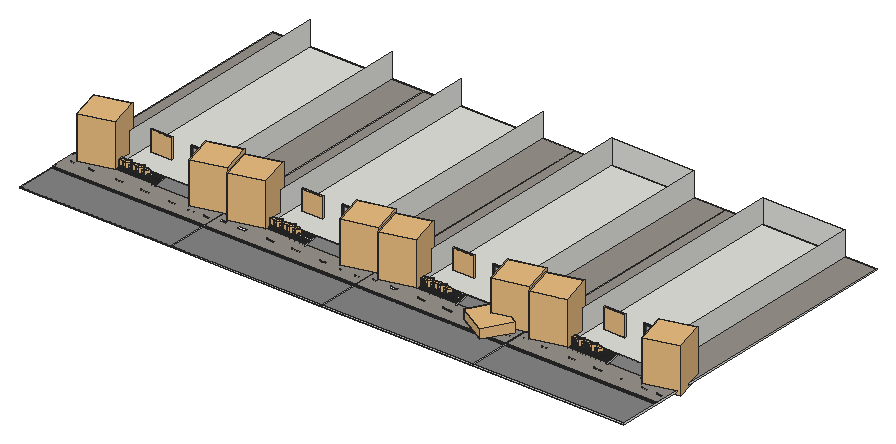
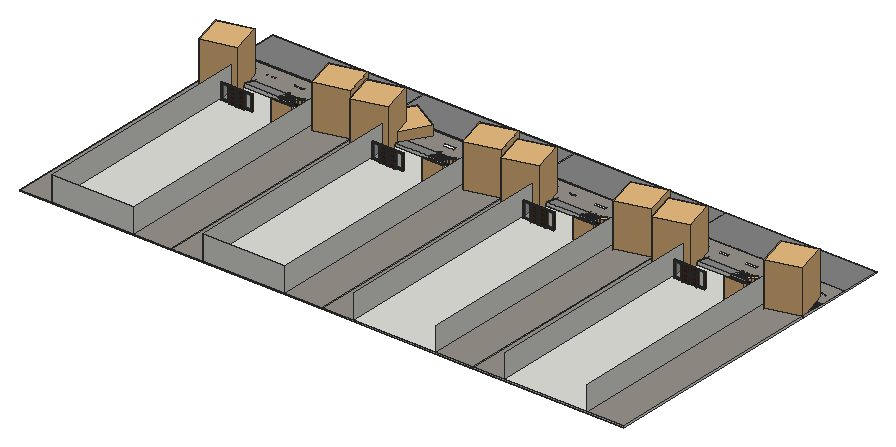
# SketchUp Ruby script. Lengths in inches.
U = 1.inch
M = Sketchup.active_model
def pt(a) = Geom::Point3d.new(a.map { |v| v * U })
def face(e, loops, mat)
  f = e.add_face(loops[0].map { |a| pt(a) })
  loops[1..].each { |l| e.add_face(l.map { |a| pt(a) }).erase! }
  f.material = f.back_material = mat if mat
  f
end
# faces: each face lists its corners as indices into pts; further lists are holes
def faces(e, pts, list, mat = nil) = list.each { |f| face(e, (f[0].is_a?(Array) ? f : [f]).map { |l| l.map { |i| pts[i] } }, mat) }
# xy, xz, yz: faces in a plane at the given z, y or x. An outline is a flat list of corners, or four numbers for a rectangle; further outlines are holes
def ring(l) = l.size == 4 ? [[l[0], l[1]], [l[2], l[1]], [l[2], l[3]], [l[0], l[3]]] : l.each_slice(2).to_a
def flat(e, list, mat, &to3) = list.each { |f| face(e, (f[0].is_a?(Array) ? f : [f]).map { |l| ring(l).map { |u, v| to3.(u, v) } }, mat) }
def xy(e, z, list, mat = nil) = flat(e, list, mat) { |x, y| [x, y, z] }
def xz(e, y, list, mat = nil) = flat(e, list, mat) { |x, z| [x, y, z] }
def yz(e, x, list, mat = nil) = flat(e, list, mat) { |y, z| [x, y, z] }
def lines(e, pts, list) = list.each { |a, b| e.add_line(pt(pts[a]), pt(pts[b])) }
# prism: a flat outline (further loops are holes) pulled along v
def prism(e, loops, v, mat = nil)
  f = face(e, loops, mat); d = Geom::Vector3d.new(v.map { |x| x * U })
  f.pushpull(f.normal.samedirection?(d) ? d.length : -d.length)
end
def box(e, o, s, mat = nil) = prism(e, [[o, [o[0] + s[0], o[1], o[2]], [o[0] + s[0], o[1] + s[1], o[2]], [o[0], o[1] + s[1], o[2]]]], [0, 0, s[2]], mat)
def at(x, y, z, deg = 0) = Geom::Transformation.translation(pt([x, y, z])) * Geom::Transformation.rotation(ORIGIN, Z_AXIS, deg.degrees)
def axes(o, x, y, z) = Geom::Transformation.new([*x, 0, *y, 0, *z, 0, *pt(o).to_a, 1])
def part(name) = M.definitions.add(name)
# library, detail: a bought-in or finely detailed component or shape, given as its bounding box
def library(name, o, s) = part(name).tap { |d| box(d.entities, o, s) }
def detail(e, o, s) = box(e.add_group.entities, o, s)
def put(e, d, t, mat = nil) = e.add_instance(d, t).tap { |i| i.material = mat if mat }
def group(e, t, mat = nil) = e.add_group.tap { |g| g.transformation = t; g.material = mat if mat }.entities
root = M.entities
M.materials.add("Color_000").color = [255, 255, 255]
M.materials.add("MADEIRAS PORTAS MOD 4").color = [48, 37, 30]
M.materials.add("Material__1").color = [95, 70, 46]
M.materials.add("[Aluminum]").color = [179, 179, 179]
M.materials.add("[Color M07]").color = [58, 58, 58]
M.materials.add("[Color M08]").color = [30, 30, 30]
M.materials.add("[Granite Dark Gray]").color = [38, 37, 37]
M.materials.add("[Granite Tile]").color = [153, 146, 141]
M.materials.add("[Tile Grey]").color = [132, 132, 132]
M.materials.add("[Tile Grey]1").color = [133, 133, 133]
M.materials.add("[Translucent Glass Gray]").color = [128, 128, 128]
M.materials["[Translucent Glass Gray]"].alpha = 0.5
M.materials.add("[Wood Veneer 01]").color = [66, 38, 20]
c1 = library("002+Bmw+M4+++mat3.4+2017",[-252.8,19.48,9.01],[196.94,171.32,55.15])
c2 = part("Untitled (5)")
xy(c2.entities,0,[[[158.81,26.5625,306.06,993.3125],[226.57,518.17,239.57,583.92],[225.28,357.51,237.28,411.51],[222.61,182.28,236.36,226.53],[239.71,931.55,251.46,972.3],[233.64,703.93,242.14,755.18],[240.05,835.03,248.8,880.53],[222.04,66.5,231.29,100.5]]])
xy(c2.entities,0,[[222.04,66.5,231.29,100.5],[222.61,182.28,236.36,226.53],[225.28,357.51,237.28,411.51],[226.57,518.17,239.57,583.92],[233.64,703.93,242.14,755.18],
  [240.05,835.03,248.8,880.53],[239.71,931.55,251.46,972.3]],"Color_000")
c3 = library("Areca palm plant",[0,0,0],[49.1,36.6,54.46])
c4 = library("Group\#74",[-84.69,-90.07,-0.36],[176.51,175.13,171.4])
c5 = library("Group38\#2",[14.01,28.44,-23.43],[18.58,18.32,38.89])
c6 = library("Group\#130",[-7.34,-1.2,0],[38.67,35.81,49.04])
c7 = library("Group20\#1",[-20.81,-17.08,3.79],[39.86,39.43,37.51])
c8 = part("Group\#3")
xy(c8.entities,0,[[0,0,6,234.8],[30,0,36,234.8]])
xy(c8.entities,3,[[6,0,30,234.8]])
xy(c8.entities,7,[[6,5,30,229.8]],"Material__1")
xy(c8.entities,15,[[[0,0,36,234.8],[6,5,30,229.8]]])
xz(c8.entities,0,[[0,0,6,0,6,3,30,3,30,0,36,0,36,15,0,15]])
xz(c8.entities,5,[[6,7,30,15]])
xz(c8.entities,229.8,[[6,7,30,15]])
xz(c8.entities,234.8,[[0,0,0,15,36,15,36,0,30,0,30,3,6,3,6,0]])
yz(c8.entities,0,[[0,0,234.8,15]])
yz(c8.entities,6,[[0,0,234.8,3],[5,7,229.8,15]])
yz(c8.entities,30,[[0,0,234.8,3],[5,7,229.8,15]])
yz(c8.entities,36,[[0,0,234.8,15]])
c9 = part("Planted trough")
put(c9.entities,c3,axes([-6.2,158.41,6.08],[0.45017,-0.56191,0],[0.66137,0.52986,0],[0,0,0.72]))
put(c9.entities,c3,axes([-6.2,56.6,6.08],[0.45017,-0.56191,0],[0.66137,0.52986,0],[0,0,0.72]))
put(c9.entities,c4,axes([17.19,15.79,6.07],[-0.08133,-0.14087,0],[0.14087,-0.08133,0],[0,0,0.1725]))
put(c9.entities,c4,axes([14.93,173.12,6.05],[-0.04961,-0.08593,0],[0.08593,-0.04961,0],[0,0,0.10522]))
put(c9.entities,c4,axes([17.19,223.04,6.07],[-0.08133,-0.14087,0],[0.14087,-0.08133,0],[0,0,0.1725]))
put(c9.entities,c5,axes([-4.1,-1.15,28.17],[0.8848,0,0],[0,0.94674,0],[0,0,0.85826]))
put(c9.entities,c4,axes([14.93,193.18,6.05],[-0.04961,-0.08593,0],[0.08593,-0.04961,0],[0,0,0.10522]))
put(c9.entities,c4,axes([14.93,91.37,6.05],[-0.04961,-0.08593,0],[0.08593,-0.04961,0],[0,0,0.10522]))
put(c9.entities,c6,axes([24.9375,191.72,8],[0,0.79,0],[-0.79,0,0],[0,0,0.79]))
put(c9.entities,c7,axes([18.97,181.79,4.77],[0,0.85,0],[-0.85,0,0],[0,0,0.85]))
put(c9.entities,c4,axes([14.93,145.87,6.05],[-0.04961,-0.08593,0],[0.08593,-0.04961,0],[0,0,0.10522]))
put(c9.entities,c7,axes([18.97,79.98,4.77],[0,0.85,0],[-0.85,0,0],[0,0,0.85]))
put(c9.entities,c4,axes([14.93,71.3,6.05],[-0.04961,-0.08593,0],[0.08593,-0.04961,0],[0,0,0.10522]))
put(c9.entities,c6,axes([24.9375,89.91,8],[0,0.79,0],[-0.79,0,0],[0,0,0.79]))
put(c9.entities,c4,axes([14.93,44.05,6.05],[-0.04961,-0.08593,0],[0.08593,-0.04961,0],[0,0,0.10522]))
put(c9.entities,c4,axes([17.19,121.23,6.07],[-0.08133,-0.14087,0],[0.14087,-0.08133,0],[0,0,0.1725]))
put(c9.entities,c8,at(0,0,0),"[Color M07]")
put(c9.entities,c5,axes([-4.1,100.66,28.17],[0.8848,0,0],[0,0.94674,0],[0,0,0.85826]))
c10 = library("Palm tree",[-4.09,-4.52,0],[193.52,193.51,258.93])
c11 = part("Palm+Tree")
put(c11.entities,c10,at(25.51,-21.81,0,15))
c12 = library("Curtains",[0,0,0],[121.73,8.19,117.22])
c13 = part("Component\#9")
prism(c13.entities,[[[23.23,0,0],[0,0,0],[0,0,74.02],[23.23,0,74.02]],[[2.76,0,2.76],[20.47,0,2.76],[20.47,0,71.26],[3.07,0,71.26]]],[0,1.38,0],"[Wood Veneer 01]")
c14 = part("Component\#1")
g1 = group(c14.entities,at(20.87,-0.79,28.35))
xy(g1,0,[[0,0,1.18,0.79]],"[Aluminum]")
xy(g1,23.62,[[0,0,1.18,0.79]],"[Aluminum]")
xz(g1,0,[[0,0,1.18,23.62]],"MADEIRAS PORTAS MOD 4")
xz(g1,0.79,[[0,0,1.18,23.62]],"[Aluminum]")
yz(g1,0,[[0,0,0.79,23.62]],"[Aluminum]")
yz(g1,1.18,[[0,0,0.79,23.62]],"[Aluminum]")
g2 = group(c14.entities,at(0,0,0),"MADEIRAS PORTAS MOD 4")
xy(g2,0,[[0,0,23.62,1.57]],"[Wood Veneer 01]")
xy(g2,80.31,[[0,0,23.62,1.57]],"[Wood Veneer 01]")
xz(g2,0,[[0,0,17.32,19.78],[17.32,0,17.32,19.78,0,19.78,0,20.18,17.32,20.18,17.32,39.96,0,39.96,0,40.35,17.32,40.35,17.32,60.14,0,60.14,0,60.53,17.32,60.53,17.32,80.31,17.72,80.31,17.72,0],[17.72,0,23.62,80.31],[0,20.18,17.32,39.96],[0,40.35,17.32,60.14],
  [0,60.53,17.32,80.31]],"[Wood Veneer 01]")
xz(g2,1.57,[[0,0,17.32,19.78],[17.32,0,17.72,0,17.72,80.31,17.32,80.31,17.32,60.53,0,60.53,0,60.14,17.32,60.14,17.32,40.35,0,40.35,0,39.96,17.32,39.96,17.32,20.18,0,20.18,0,19.78,17.32,19.78],[17.72,0,23.62,80.31],[0,20.18,17.32,39.96],[0,40.35,17.32,60.14],
  [0,60.53,17.32,80.31]],"[Wood Veneer 01]")
yz(g2,0,[[0,0,1.57,80.31]],"[Wood Veneer 01]")
yz(g2,23.62,[[0,0,1.57,80.31]],"[Wood Veneer 01]")
g3 = group(c14.entities,at(20.87,2.36,28.35))
box(g3,[0,-0.79,0],[1.18,0.79,23.62],"[Aluminum]")
c15 = part("Component\#8")
xz(c15.entities,2.95,[[-20.47,9.06,-2.76,77.56],[54.72,9.06,72.44,77.56]],"[Translucent Glass Gray]")
put(c15.entities,c13,at(-23.23,2.26,6.3),"MADEIRAS PORTAS MOD 4")
put(c15.entities,c13,axes([75.2,2.26,6.3],[-1,0,0],[0,1,0],[0,0,1]))
put(c15.entities,c14,at(2.36,2.17,0),"MADEIRAS PORTAS MOD 4")
put(c15.entities,c14,axes([49.61,2.17,0],[-1,0,0],[0,1,0],[0,0,1]))
g4 = group(c15.entities,at(0,0,0),"MADEIRAS PORTAS MOD 4")
xy(g4,0,[[0,0,2.36,5.91],[49.61,0,51.97,5.91]],"[Wood Veneer 01]")
xy(g4,3.9375,[[-25.59,0,0,5.91],[51.97,0,77.56,5.91]],"[Wood Veneer 01]")
xy(g4,6.3,[[-23.23,0,0,5.91],[51.97,0,75.2,5.91]],"[Wood Veneer 01]")
xy(g4,80.31,[[-23.23,0,0,5.91],[2.36,0,49.61,5.91],[51.97,0,75.2,5.91]],"[Wood Veneer 01]")
xy(g4,82.68,[[-25.59,0,77.56,5.91]],"[Wood Veneer 01]")
xz(g4,0,[[[0,0,2.36,0,2.36,80.31,49.61,80.31,49.61,0,51.97,0,51.97,3.9375,77.56,3.9375,77.56,82.68,-25.59,82.68,-25.59,3.9375,0,3.9375,0,6.3,-23.23,6.3,-23.23,80.31,0,80.31],[51.97,6.3,75.2,80.31]]],"MADEIRAS PORTAS MOD 4")
xz(g4,5.91,[[[0,0,2.36,0,2.36,80.31,49.61,80.31,49.61,0,51.97,0,51.97,3.9375,77.56,3.9375,77.56,82.68,-25.59,82.68,-25.59,3.9375,0,3.9375,0,6.3,-23.23,6.3,-23.23,80.31,0,80.31],[51.97,6.3,75.2,80.31]]],"[Wood Veneer 01]")
yz(g4,-25.59,[[0,3.9375,5.91,82.68]],"[Wood Veneer 01]")
yz(g4,-23.23,[[0,6.3,5.91,80.31]],"[Wood Veneer 01]")
yz(g4,0,[[0,0,5.91,3.9375],[0,3.9375,5.91,6.3],[0,6.3,5.91,80.31]],"[Wood Veneer 01]")
yz(g4,2.36,[[0,0,5.91,80.31]],"[Wood Veneer 01]")
yz(g4,49.61,[[0,0,5.91,80.31]],"[Wood Veneer 01]")
yz(g4,51.97,[[0,0,5.91,3.9375],[0,3.9375,5.91,6.3],[0,6.3,5.91,80.31]],"[Wood Veneer 01]")
yz(g4,75.2,[[0,6.3,5.91,80.31]],"[Wood Veneer 01]")
yz(g4,77.56,[[0,3.9375,5.91,82.68]],"[Wood Veneer 01]")
c16 = part("Wood+Door (2)")
put(c16.entities,c15,at(25.59,0,0),"MADEIRAS PORTAS MOD 4")
xy(root,-18.8125,[[1.85,0,880.6,1835.625],[880.6,0,1759.35,1835.625],[1759.35,0,2638.1,1835.625],[2638.1,0,3516.85,1835.625]])
xy(root,-13.3125,[[395.95,428.3125,463.7,438.375],[1274.7,428.3125,1342.45,438.375],[2153.45,428.3125,2221.2,438.375],[3032.2,428.3125,3099.95,438.375],[395.95,438.375,463.7,450],
  [1274.7,438.375,1342.45,450],[2153.45,438.375,2221.2,450],[3032.2,438.375,3099.95,450]])
xy(root,-11.3125,[[480.15,370.25,678.9,370.25,678.9,458.5,493.86,458.5,493.86,382.55,480.15,382.55],[1358.9,370.25,1557.65,370.25,1557.65,458.5,1372.61,458.5,1372.61,382.55,1358.9,382.55],[2237.65,370.25,2436.4,370.25,2436.4,458.5,2251.36,458.5,2251.36,382.55,2237.65,382.55],[3116.4,370.25,3315.15,370.25,3315.15,458.5,3130.11,458.5,3130.11,382.55,3116.4,382.55],[479.03,382.55,480.15,428.3125],
  [480.15,382.55,493.86,458.5],[1357.78,382.55,1358.9,428.3125],[1358.9,382.55,1372.61,458.5],[2236.53,382.55,2237.65,428.3125],[2237.65,382.55,2251.36,458.5],
  [3115.28,382.55,3116.4,428.3125],[3116.4,382.55,3130.11,458.5],[463.7,428.3125,479.03,438.375],[479.03,428.3125,480.15,438.375],[1342.45,428.3125,1357.78,438.375],
  [1357.78,428.3125,1358.9,438.375],[2221.2,428.3125,2236.53,438.375],[2236.53,428.3125,2237.65,438.375],[3099.95,428.3125,3115.28,438.375],[3115.28,428.3125,3116.4,438.375],
  [463.7,438.375,479.03,450],[479.03,438.375,480.15,450],[1342.45,438.375,1357.78,450],[1357.78,438.375,1358.9,450],[2221.2,438.375,2236.53,450],
  [2236.53,438.375,2237.65,450],[3099.95,438.375,3115.28,450],[3115.28,438.375,3116.4,450],[479.03,450,480.15,450,480.15,458.5,698.16,458.5,698.16,1835.625,218.97,1835.625,218.97,458.5,479.03,458.5],[1357.78,450,1358.9,450,1358.9,458.5,1576.91,458.5,1576.91,1835.625,1097.72,1835.625,1097.72,458.5,1357.78,458.5],
  [2236.53,450,2237.65,450,2237.65,458.5,2455.66,458.5,2455.66,1835.625,1976.47,1835.625,1976.47,458.5,2236.53,458.5],[3115.28,450,3116.4,450,3116.4,458.5,3334.41,458.5,3334.41,1835.625,2855.22,1835.625,2855.22,458.5,3115.28,458.5]])
xy(root,-11.3125,[[1.85,226.76,880.6,226.76,880.6,458.5,678.9,458.5,678.9,370.25,480.15,370.25,480.15,382.55,1.85,382.55],[880.6,226.76,1759.35,226.76,1759.35,458.5,1557.65,458.5,1557.65,370.25,1358.9,370.25,1358.9,382.55,880.6,382.55],[1759.35,226.76,2638.1,226.76,2638.1,458.5,2436.4,458.5,2436.4,370.25,2237.65,370.25,2237.65,382.55,1759.35,382.55],[2638.1,226.76,3516.85,226.76,3516.85,458.5,3315.15,458.5,3315.15,370.25,3116.4,370.25,3116.4,382.55,2638.1,382.55]],"[Granite Dark Gray]")
xy(root,-11.3125,[[1.85,458.5,218.97,1835.625],[698.16,458.5,880.6,1835.625],[880.6,458.5,1097.72,1835.625],[1576.91,458.5,1759.35,1835.625],[1759.35,458.5,1976.47,1835.625],
  [2455.66,458.5,2638.1,1835.625],[2638.1,458.5,2855.22,1835.625],[3334.41,458.5,3516.85,1835.625]],"[Granite Tile]")
xy(root,-11.3125,[[1.85,0,880.6,226.76],[880.6,0,1759.35,226.76],[1759.35,0,2638.1,226.76],[2638.1,0,3516.85,226.76]],"[Tile Grey]1")
xy(root,-9.1875,[[1.85,382.55,479.03,458.5],[880.6,382.55,1357.78,458.5],[1759.35,382.55,2236.53,458.5],[2638.1,382.55,3115.28,458.5]],"[Granite Dark Gray]")
xy(root,-7.25,[[395.95,438.375,480.15,450],[1274.7,438.375,1358.9,450],[2153.45,438.375,2237.65,450],[3032.2,438.375,3116.4,450],[395.95,450,480.15,458.5],
  [1274.7,450,1358.9,458.5],[2153.45,450,2237.65,458.5],[3032.2,450,3116.4,458.5]])
xy(root,-3.25,[[395.95,428.3125,480.15,438.375],[1274.7,428.3125,1358.9,438.375],[2153.45,428.3125,2237.65,438.375],[3032.2,428.3125,3116.4,438.375]])
xy(root,0,[[395.95,450,480.15,458.5],[1274.7,450,1358.9,458.5],[2153.45,450,2237.65,458.5],[3032.2,450,3116.4,458.5]])
xy(root,3.25,[[395.95,438.375,480.15,450],[1274.7,438.375,1358.9,450],[2153.45,438.375,2237.65,450],[3032.2,438.375,3116.4,450]])
xz(root,0,[[1.85,-18.8125,880.6,-11.3125],[880.6,-18.8125,1759.35,-11.3125],[1759.35,-18.8125,2638.1,-11.3125],[2638.1,-18.8125,3516.85,-11.3125]])
xz(root,382.55,[[1.85,-11.3125,379.41,-9.1875],[379.41,-11.3125,479.03,-9.1875],[479.03,-11.3125,493.86,-11.3125,479.03,-9.1875],[880.6,-11.3125,1258.16,-9.1875],[1258.16,-11.3125,1357.78,-9.1875],
  [1357.78,-11.3125,1372.61,-11.3125,1357.78,-9.1875],[1759.35,-11.3125,2136.91,-9.1875],[2136.91,-11.3125,2236.53,-9.1875],[2236.53,-11.3125,2251.36,-11.3125,2236.53,-9.1875],[2638.1,-11.3125,3015.66,-9.1875],
  [3015.66,-11.3125,3115.28,-9.1875],[3115.28,-11.3125,3130.11,-11.3125,3115.28,-9.1875]])
xz(root,428.3125,[[395.95,-13.3125,463.7,-13.3125,463.7,-11.3125,480.15,-11.3125,480.15,-3.25,395.95,-3.25],[1274.7,-13.3125,1342.45,-13.3125,1342.45,-11.3125,1358.9,-11.3125,1358.9,-3.25,1274.7,-3.25],[2153.45,-13.3125,2221.2,-13.3125,2221.2,-11.3125,2237.65,-11.3125,2237.65,-3.25,2153.45,-3.25],[3032.2,-13.3125,3099.95,-13.3125,3099.95,-11.3125,3116.4,-11.3125,3116.4,-3.25,3032.2,-3.25]],"[Color M08]")
xz(root,438.375,[[395.95,-7.25,480.15,-3.25],[1274.7,-7.25,1358.9,-3.25],[2153.45,-7.25,2237.65,-3.25],[3032.2,-7.25,3116.4,-3.25]])
xz(root,438.375,[[395.95,-3.25,480.15,3.25],[1274.7,-3.25,1358.9,3.25],[2153.45,-3.25,2237.65,3.25],[3032.2,-3.25,3116.4,3.25]],"[Color M08]")
xz(root,450,[[395.95,-13.3125,395.95,-7.25,480.15,-7.25,480.15,-11.3125,463.7,-11.3125,463.7,-13.3125],[1274.7,-13.3125,1274.7,-7.25,1358.9,-7.25,1358.9,-11.3125,1342.45,-11.3125,1342.45,-13.3125],[2153.45,-13.3125,2153.45,-7.25,2237.65,-7.25,2237.65,-11.3125,2221.2,-11.3125,2221.2,-13.3125],[3032.2,-13.3125,3032.2,-7.25,3116.4,-7.25,3116.4,-11.3125,3099.95,-11.3125,3099.95,-13.3125],[395.95,0,480.15,3.25],
  [1274.7,0,1358.9,3.25],[2153.45,0,2237.65,3.25],[3032.2,0,3116.4,3.25]])
xz(root,450,[[395.95,3.25,480.15,8.5],[1274.7,3.25,1358.9,8.5],[2153.45,3.25,2237.65,8.5],[3032.2,3.25,3116.4,8.5]],"[Color M08]")
xz(root,458.5,[[1.85,-11.3125,218.97,-9.1875],[218.97,-11.3125,395.95,-9.1875],[395.95,-11.3125,463.7,-9.1875],[463.7,-11.3125,479.03,-9.1875],[480.15,-11.3125,480.15,-9.35,493.86,-11.3125],
  [493.86,-11.3125,678.9,-11.3125,678.9,8.5,480.15,8.5,480.15,-9.35],[880.6,-11.3125,1097.72,-9.1875],[1097.72,-11.3125,1274.7,-9.1875],[1274.7,-11.3125,1342.45,-9.1875],[1342.45,-11.3125,1357.78,-9.1875],
  [1358.9,-11.3125,1358.9,-9.35,1372.61,-11.3125],[1372.61,-11.3125,1557.65,-11.3125,1557.65,8.5,1358.9,8.5,1358.9,-9.35],[1759.35,-11.3125,1976.47,-9.1875],[1976.47,-11.3125,2153.45,-9.1875],[2153.45,-11.3125,2221.2,-9.1875],
  [2221.2,-11.3125,2236.53,-9.1875],[2237.65,-11.3125,2237.65,-9.35,2251.36,-11.3125],[2251.36,-11.3125,2436.4,-11.3125,2436.4,8.5,2237.65,8.5,2237.65,-9.35],[2638.1,-11.3125,2855.22,-9.1875],[2855.22,-11.3125,3032.2,-9.1875],
  [3032.2,-11.3125,3099.95,-9.1875],[3099.95,-11.3125,3115.28,-9.1875],[3116.4,-11.3125,3116.4,-9.35,3130.11,-11.3125],[3130.11,-11.3125,3315.15,-11.3125,3315.15,8.5,3116.4,8.5,3116.4,-9.35],[395.95,-9.1875,463.7,-7.25],
  [1274.7,-9.1875,1342.45,-7.25],[2153.45,-9.1875,2221.2,-7.25],[3032.2,-9.1875,3099.95,-7.25],[395.95,-7.25,480.15,0],[1274.7,-7.25,1358.9,0],
  [2153.45,-7.25,2237.65,0],[3032.2,-7.25,3116.4,0],[395.95,0,480.15,8.5],[1274.7,0,1358.9,8.5],[2153.45,0,2237.65,8.5],
  [3032.2,0,3116.4,8.5]])
xz(root,458.5,[[480.15,-9.35,480.15,-7.25,463.7,-7.25,463.7,-9.1875,479.03,-9.1875],[1358.9,-9.35,1358.9,-7.25,1342.45,-7.25,1342.45,-9.1875,1357.78,-9.1875],[2237.65,-9.35,2237.65,-7.25,2221.2,-7.25,2221.2,-9.1875,2236.53,-9.1875],[3116.4,-9.35,3116.4,-7.25,3099.95,-7.25,3099.95,-9.1875,3115.28,-9.1875]],"[Color M07]")
xz(root,458.5,[[218.97,-9.1875,395.95,8.5],[1097.72,-9.1875,1274.7,8.5],[1976.47,-9.1875,2153.45,8.5],[2855.22,-9.1875,3032.2,8.5]],"[Color M08]")
xz(root,458.5,[[678.9,-11.3125,698.16,118.38],[1557.65,-11.3125,1576.91,118.38],[2436.4,-11.3125,2455.66,118.38],[3315.15,-11.3125,3334.41,118.38]],"[Wood Veneer 01]")
xz(root,1835.625,[[1.85,-18.8125,880.6,-11.3125],[880.6,-18.8125,1759.35,-11.3125],[1759.35,-18.8125,2638.1,-11.3125],[2638.1,-18.8125,3516.85,-11.3125],[1976.47,-11.3125,2455.66,128.5],
  [2855.22,-11.3125,3334.41,128.5]])
yz(root,1.85,[[0,-18.8125,0,-11.3125,382.55,-11.3125,382.55,-9.1875,458.5,-9.1875,458.5,-11.3125,1835.625,-11.3125,1835.625,-18.8125]])
yz(root,218.97,[[458.5,-11.3125,458.5,8.5,523.18,8.5,523.18,128.5,1835.625,128.5,1835.625,-11.3125]])
yz(root,395.95,[[428.3125,-13.3125,438.375,-11.3125],[438.375,-13.3125,450,-11.3125],[428.3125,-11.3125,438.375,-3.25],[438.375,-11.3125,450,-7.25],[438.375,-7.25,450,3.25],
  [450,-7.25,458.5,0],[450,0,458.5,8.5]])
yz(root,463.7,[[428.3125,-13.3125,438.375,-11.3125],[438.375,-13.3125,450,-11.3125]])
yz(root,479.03,[[382.55,-11.3125,458.5,-9.1875]])
yz(root,480.15,[[370.25,-11.3125,450,6.59,450,3.25,438.375,3.25,438.375,-3.25,428.3125,-3.25,428.3125,-11.3125],[428.3125,-11.3125,450,-11.3125,450,-7.25,438.375,-7.25,438.375,-3.25,428.3125,-3.25],[450,-11.3125,458.5,-7.25],[450,0,450,6.59,458.5,8.5,458.5,0],[450,6.59,458.5,8.5,450,8.5]])
yz(root,678.9,[[370.25,-11.3125,458.5,-11.3125,458.5,8.5]])
yz(root,698.16,[[458.5,-11.3125,1835.625,128.5]])
yz(root,880.6,[[0,-18.8125,1835.625,-11.3125],[382.55,-11.3125,458.5,-9.1875]])
yz(root,1097.72,[[458.5,-11.3125,458.5,8.5,523.18,8.5,523.18,128.5,1835.625,128.5,1835.625,-11.3125]])
yz(root,1274.7,[[428.3125,-13.3125,438.375,-11.3125],[438.375,-13.3125,450,-11.3125],[428.3125,-11.3125,438.375,-3.25],[438.375,-11.3125,450,-7.25],[438.375,-7.25,450,3.25],
  [450,-7.25,458.5,0],[450,0,458.5,8.5]])
yz(root,1342.45,[[428.3125,-13.3125,438.375,-11.3125],[438.375,-13.3125,450,-11.3125]])
yz(root,1357.78,[[382.55,-11.3125,458.5,-9.1875]])
yz(root,1358.9,[[370.25,-11.3125,450,6.59,450,3.25,438.375,3.25,438.375,-3.25,428.3125,-3.25,428.3125,-11.3125],[428.3125,-11.3125,450,-11.3125,450,-7.25,438.375,-7.25,438.375,-3.25,428.3125,-3.25],[450,-11.3125,458.5,-7.25],[450,0,450,6.59,458.5,8.5,458.5,0],[450,6.59,458.5,8.5,450,8.5]])
yz(root,1557.65,[[370.25,-11.3125,458.5,-11.3125,458.5,8.5]])
yz(root,1576.91,[[458.5,-11.3125,1835.625,128.5]])
yz(root,1759.35,[[0,-18.8125,1835.625,-11.3125],[382.55,-11.3125,458.5,-9.1875]])
yz(root,1976.47,[[458.5,-11.3125,458.5,8.5,523.18,8.5,523.18,128.5,1835.625,128.5,1835.625,-11.3125]])
yz(root,2153.45,[[428.3125,-13.3125,438.375,-11.3125],[438.375,-13.3125,450,-11.3125],[428.3125,-11.3125,438.375,-3.25],[438.375,-11.3125,450,-7.25],[438.375,-7.25,450,3.25],
  [450,-7.25,458.5,0],[450,0,458.5,8.5]])
yz(root,2221.2,[[428.3125,-13.3125,438.375,-11.3125],[438.375,-13.3125,450,-11.3125]])
yz(root,2236.53,[[382.55,-11.3125,458.5,-9.1875]])
yz(root,2237.65,[[370.25,-11.3125,450,6.59,450,3.25,438.375,3.25,438.375,-3.25,428.3125,-3.25,428.3125,-11.3125],[428.3125,-11.3125,450,-11.3125,450,-7.25,438.375,-7.25,438.375,-3.25,428.3125,-3.25],[450,-11.3125,458.5,-7.25],[450,0,450,6.59,458.5,8.5,458.5,0],[450,6.59,458.5,8.5,450,8.5]])
yz(root,2436.4,[[370.25,-11.3125,458.5,-11.3125,458.5,8.5]])
yz(root,2455.66,[[458.5,-11.3125,1835.625,128.5]])
yz(root,2638.1,[[0,-18.8125,1835.625,-11.3125],[382.55,-11.3125,458.5,-9.1875]])
yz(root,2855.22,[[458.5,-11.3125,458.5,8.5,523.18,8.5,523.18,128.5,1835.625,128.5,1835.625,-11.3125]])
yz(root,3032.2,[[428.3125,-13.3125,438.375,-11.3125],[438.375,-13.3125,450,-11.3125],[428.3125,-11.3125,438.375,-3.25],[438.375,-11.3125,450,-7.25],[438.375,-7.25,450,3.25],
  [450,-7.25,458.5,0],[450,0,458.5,8.5]])
yz(root,3099.95,[[428.3125,-13.3125,438.375,-11.3125],[438.375,-13.3125,450,-11.3125]])
yz(root,3115.28,[[382.55,-11.3125,458.5,-9.1875]])
yz(root,3116.4,[[370.25,-11.3125,450,6.59,450,3.25,438.375,3.25,438.375,-3.25,428.3125,-3.25,428.3125,-11.3125],[428.3125,-11.3125,450,-11.3125,450,-7.25,438.375,-7.25,438.375,-3.25,428.3125,-3.25],[450,-11.3125,458.5,-7.25],[450,0,450,6.59,458.5,8.5,458.5,0],[450,6.59,458.5,8.5,450,8.5]])
yz(root,3315.15,[[370.25,-11.3125,458.5,-11.3125,458.5,8.5]])
yz(root,3334.41,[[458.5,-11.3125,1835.625,128.5]])
yz(root,3516.85,[[0,-18.8125,1835.625,-11.3125]])
p = [[678.9,370.25,-11.3125],[678.9,458.5,8.5],[481.29,458.5,8.5],[480.15,458.5,8.5],[480.15,450,6.59],[480.15,370.25,-11.3125],
  [1557.65,370.25,-11.3125],[1557.65,458.5,8.5],[1360.04,458.5,8.5],[1358.9,458.5,8.5],[1358.9,450,6.59],[1358.9,370.25,-11.3125],
  [2436.4,370.25,-11.3125],[2436.4,458.5,8.5],[2238.79,458.5,8.5],[2237.65,458.5,8.5],[2237.65,450,6.59],[2237.65,370.25,-11.3125],
  [3315.15,370.25,-11.3125],[3315.15,458.5,8.5],[3117.54,458.5,8.5],[3116.4,458.5,8.5],[3116.4,450,6.59],[3116.4,370.25,-11.3125],
  [480.15,458.5,-9.35],[479.03,458.5,-9.1875],[479.03,382.55,-9.1875],[493.86,382.55,-11.3125],[493.86,458.5,-11.3125],[1358.9,458.5,-9.35],
  [1357.78,458.5,-9.1875],[1357.78,382.55,-9.1875],[1372.61,382.55,-11.3125],[1372.61,458.5,-11.3125],[2237.65,458.5,-9.35],[2236.53,458.5,-9.1875],
  [2236.53,382.55,-9.1875],[2251.36,382.55,-11.3125],[2251.36,458.5,-11.3125],[3116.4,458.5,-9.35],[3115.28,458.5,-9.1875],[3115.28,382.55,-9.1875],
  [3130.11,382.55,-11.3125],[3130.11,458.5,-11.3125],[2221.2,458.5,-11.3125],[2221.2,450,-11.3125],[2153.45,458.5,-11.3125],[2153.45,450,-11.3125],
  [3099.95,458.5,-11.3125],[3099.95,450,-11.3125],[3032.2,458.5,-11.3125],[3032.2,450,-11.3125],[463.7,458.5,-11.3125],[463.7,450,-11.3125],
  [395.95,458.5,-11.3125],[395.95,450,-11.3125],[1274.7,458.5,-11.3125],[1274.7,450,-11.3125],[1342.45,458.5,-11.3125],[1342.45,450,-11.3125]]
faces(root,p,[[0,1,2,3,4,5],[6,7,8,9,10,11],[12,13,14,15,16,17],[18,19,20,21,22,23]],"[Tile Grey]")
faces(root,p,[[24,25,26,27,28],[29,30,31,32,33],[34,35,36,37,38],[39,40,41,42,43]])
lines(root,p,[[44,45],[46,47],[48,49],[50,51],[52,53],[54,55],[56,57],[58,59]])
put(root,c1,at(2565.55,143.27,-11.3125,-30))
put(root,c2,axes([2612.05,547.28,-7.22],[0,-1,0],[0.91088,0,0],[0,0,1]),"[Granite Tile]")
put(root,c2,axes([-24.2,547.28,-7.22],[0,-1,0],[0.91088,0,0],[0,0,1]),"[Granite Tile]")
put(root,c2,axes([854.55,547.28,-7.22],[0,-1,0],[0.91088,0,0],[0,0,1]),"[Granite Tile]")
put(root,c2,axes([1733.3,547.28,-7.22],[0,-1,0],[0.91088,0,0],[0,0,1]),"[Granite Tile]")
put(root,c9,axes([2154.48,426.74,-7.25],[0,0.7469,0],[-0.7469,0,0],[0,0,0.7469]))
put(root,c9,axes([3033.23,426.74,-7.25],[0,0.7469,0],[-0.7469,0,0],[0,0,0.7469]))
put(root,c9,axes([1275.73,426.74,-7.25],[0,0.7469,0],[-0.7469,0,0],[0,0,0.7469]))
put(root,c9,axes([396.98,426.74,-7.25],[0,0.7469,0],[-0.7469,0,0],[0,0,0.7469]))
put(root,c11,at(2448.27,365.67,-29.65))
put(root,c11,at(3327.02,365.67,-29.65))
put(root,c11,at(1569.52,365.67,-29.65))
put(root,c11,at(690.77,365.67,-29.65))
put(root,c11,at(1789.25,369.08,-20.67))
put(root,c11,at(2668,369.08,-20.67))
put(root,c11,at(910.5,369.08,-20.67))
put(root,c11,at(31.75,369.08,-20.67))
put(root,c12,at(2022.96,623.11,-9.86))
put(root,c12,at(2901.71,623.11,-9.86))
put(root,c12,at(265.46,623.11,-9.86))
put(root,c12,at(1144.21,623.11,-9.86))
put(root,c16,axes([3125.15,633.06,0],[1.75378,0,0],[0,1,0],[0,0,1.16459]))
put(root,c16,axes([488.9,633.06,0],[1.75378,0,0],[0,1,0],[0,0,1.16459]))
put(root,c16,axes([1367.65,633.06,0],[1.75378,0,0],[0,1,0],[0,0,1.16459]))
put(root,c16,axes([2246.4,633.06,0],[1.75378,0,0],[0,1,0],[0,0,1.16459]))
